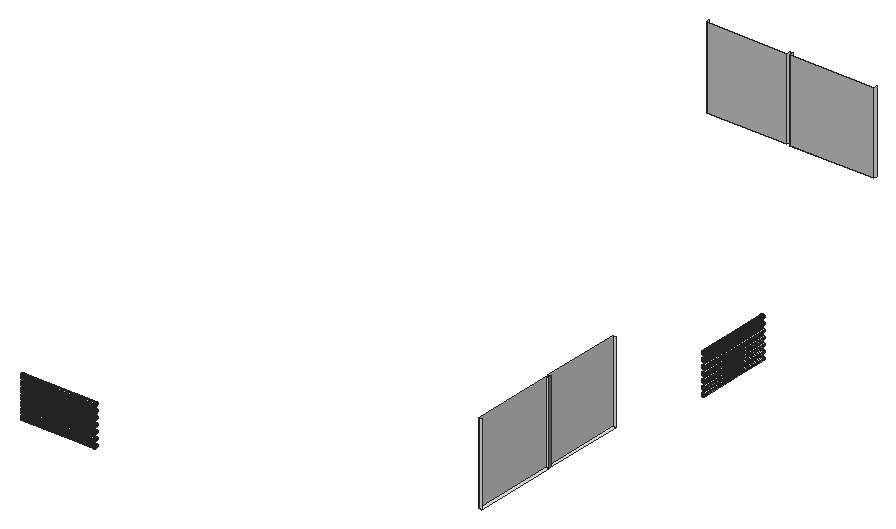
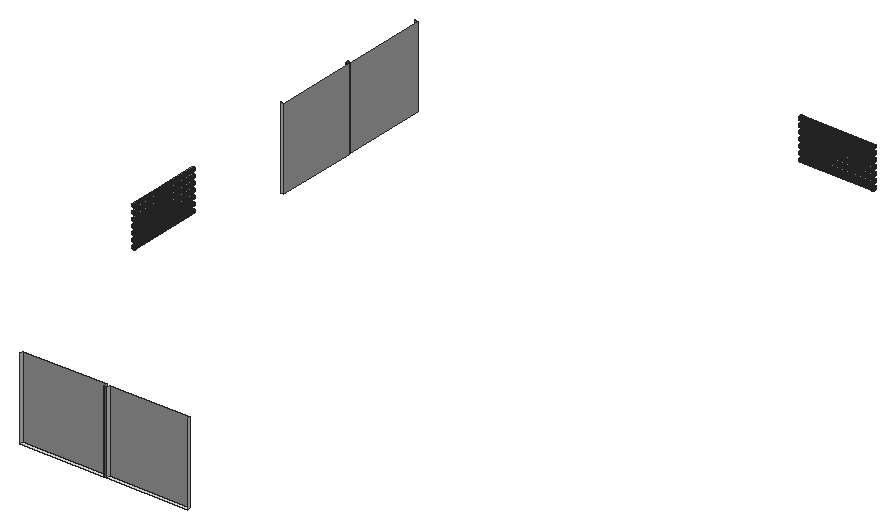
# SketchUp Ruby script. Lengths in inches.
U = 1.inch
M = Sketchup.active_model
def pt(a) = Geom::Point3d.new(a.map { |v| v * U })
def face(e, loops, mat)
  f = e.add_face(loops[0].map { |a| pt(a) })
  loops[1..].each { |l| e.add_face(l.map { |a| pt(a) }).erase! }
  f.material = f.back_material = mat if mat
  f
end
# faces: each face lists its corners as indices into pts; further lists are holes
def faces(e, pts, list, mat = nil) = list.each { |f| face(e, (f[0].is_a?(Array) ? f : [f]).map { |l| l.map { |i| pts[i] } }, mat) }
# xy, xz, yz: faces in a plane at the given z, y or x. An outline is a flat list of corners, or four numbers for a rectangle; further outlines are holes
def ring(l) = l.size == 4 ? [[l[0], l[1]], [l[2], l[1]], [l[2], l[3]], [l[0], l[3]]] : l.each_slice(2).to_a
def flat(e, list, mat, &to3) = list.each { |f| face(e, (f[0].is_a?(Array) ? f : [f]).map { |l| ring(l).map { |u, v| to3.(u, v) } }, mat) }
def xy(e, z, list, mat = nil) = flat(e, list, mat) { |x, y| [x, y, z] }
def xz(e, y, list, mat = nil) = flat(e, list, mat) { |x, z| [x, y, z] }
def yz(e, x, list, mat = nil) = flat(e, list, mat) { |y, z| [x, y, z] }
def lines(e, pts, list) = list.each { |a, b| e.add_line(pt(pts[a]), pt(pts[b])) }
# prism: a flat outline (further loops are holes) pulled along v
def prism(e, loops, v, mat = nil)
  f = face(e, loops, mat); d = Geom::Vector3d.new(v.map { |x| x * U })
  f.pushpull(f.normal.samedirection?(d) ? d.length : -d.length)
end
def box(e, o, s, mat = nil) = prism(e, [[o, [o[0] + s[0], o[1], o[2]], [o[0] + s[0], o[1] + s[1], o[2]], [o[0], o[1] + s[1], o[2]]]], [0, 0, s[2]], mat)
def at(x, y, z, deg = 0) = Geom::Transformation.translation(pt([x, y, z])) * Geom::Transformation.rotation(ORIGIN, Z_AXIS, deg.degrees)
def axes(o, x, y, z) = Geom::Transformation.new([*x, 0, *y, 0, *z, 0, *pt(o).to_a, 1])
def part(name) = M.definitions.add(name)
# library, detail: a bought-in or finely detailed component or shape, given as its bounding box
def library(name, o, s) = part(name).tap { |d| box(d.entities, o, s) }
def detail(e, o, s) = box(e.add_group.entities, o, s)
def put(e, d, t, mat = nil) = e.add_instance(d, t).tap { |i| i.material = mat if mat }
def group(e, t, mat = nil) = e.add_group.tap { |g| g.transformation = t; g.material = mat if mat }.entities
root = M.entities
M.materials.add("[Metal Seamed]").color = [118, 119, 115]
M.materials.add("[Mirror 01]").color = [185, 185, 185]
xy(root,539.76,[[1476,277.47,1482,438.75],[1476,444.75,1482,600.03],[984.78,1440.8125,1140.0625,1446.8125],[1146.0625,1440.8125,1307.35,1446.8125]])
xz(root,277.47,[[1476,539.76,1482,696.625]])
xz(root,438.75,[[1476,539.76,1482,696.625]])
xz(root,444.75,[[1476,539.76,1482,696.625]])
xz(root,600.03,[[1476,539.76,1482,696.625]])
xz(root,1440.8125,[[984.78,539.76,1140.0625,696.625],[1146.0625,539.76,1307.35,696.625]],"[Mirror 01]")
xz(root,1446.8125,[[1140.0625,539.76,1146.0625,696.625]],"[Metal Seamed]")
yz(root,984.78,[[1440.8125,539.76,1446.8125,696.625]])
yz(root,1140.0625,[[1440.8125,539.76,1446.8125,696.625]])
yz(root,1146.0625,[[1440.8125,539.76,1446.8125,696.625]])
yz(root,1307.35,[[1440.8125,539.76,1446.8125,696.625]])
yz(root,1476,[[277.47,539.76,438.75,696.625],[444.75,539.76,600.03,696.625]],"[Mirror 01]")
yz(root,1482,[[438.75,539.76,444.75,696.625]],"[Metal Seamed]")
p = [[922.01,48.34,549.02],[922.01,47.38,549.14],[778.64,47.38,549.14],[778.64,48.34,549.02],[922.01,49.29,549.14],[778.64,49.29,549.14],
  [1535.52,886.83,549.14],[1536.47,886.83,549.02],[1536.47,743.45,549.02],[1535.52,743.45,549.14],[1537.43,886.83,549.14],[1537.43,743.45,549.14],
  [922.01,46.5,549.51],[778.64,46.5,549.51],[922.01,50.18,549.51],[778.64,50.18,549.51],[1534.63,886.83,549.51],[1534.63,743.45,549.51],
  [1538.32,886.83,549.51],[1538.32,743.45,549.51],[922.01,45.73,550.1],[778.64,45.73,550.1],[922.01,50.95,550.1],[778.64,50.95,550.1],
  [1533.87,886.83,550.1],[1533.87,743.45,550.1],[1539.08,886.83,550.1],[1539.08,743.45,550.1],[922.01,45.15,550.86],[778.64,45.15,550.86],
  [922.01,51.53,550.86],[778.64,51.53,550.86],[1533.28,886.83,550.86],[1533.28,743.45,550.86],[1539.67,886.83,550.86],[1539.67,743.45,550.86],
  [922.01,44.78,551.75],[778.64,44.78,551.75],[922.01,51.9,551.75],[778.64,51.9,551.75],[1532.91,886.83,551.75],[1532.91,743.45,551.75],
  [1540.03,886.83,551.75],[1540.03,743.45,551.75],[922.01,44.65,552.7],[778.64,44.65,552.7],[922.01,52.03,552.7],[778.64,52.03,552.7],
  [1532.79,886.83,552.7],[1532.79,743.45,552.7],[1540.16,886.83,552.7],[1540.16,743.45,552.7],[922.01,44.78,553.66],[778.64,44.78,553.66],
  [922.01,51.9,553.66],[778.64,51.9,553.66],[1532.91,886.83,553.66],[1532.91,743.45,553.66],[1540.03,886.83,553.66],[1540.03,743.45,553.66],
  [922.01,45.15,554.55],[778.64,45.15,554.55],[922.01,51.53,554.55],[778.64,51.53,554.55],[1533.28,886.83,554.55],[1533.28,743.45,554.55],
  [1539.67,886.83,554.55],[1539.67,743.45,554.55],[922.01,45.73,555.3125],[778.64,45.73,555.3125],[922.01,50.95,555.3125],[778.64,50.95,555.3125],
  [1533.87,886.83,555.3125],[1533.87,743.45,555.3125],[1539.08,886.83,555.3125],[1539.08,743.45,555.3125],[922.01,46.5,555.9],[778.64,46.5,555.9],
  [922.01,50.18,555.9],[778.64,50.18,555.9],[1534.63,886.83,555.9],[1534.63,743.45,555.9],[1538.32,886.83,555.9],[1538.32,743.45,555.9],
  [922.01,47.38,556.27],[778.64,47.38,556.27],[922.01,49.29,556.27],[778.64,49.29,556.27],[1535.52,886.83,556.27],[1535.52,743.45,556.27],
  [1537.43,886.83,556.27],[1537.43,743.45,556.27],[922.01,48.34,556.39],[778.64,48.34,556.39],[1536.47,886.83,556.39],[1536.47,743.45,556.39],
  [922.01,48.34,561.02],[922.01,47.38,561.14],[778.64,47.38,561.14],[778.64,48.34,561.02],[922.01,49.29,561.14],[778.64,49.29,561.14],
  [1535.52,886.83,561.14],[1536.47,886.83,561.02],[1536.47,743.45,561.02],[1535.52,743.45,561.14],[1537.43,886.83,561.14],[1537.43,743.45,561.14],
  [922.01,46.5,561.51],[778.64,46.5,561.51],[922.01,50.18,561.51],[778.64,50.18,561.51],[1534.63,886.83,561.51],[1534.63,743.45,561.51],
  [1538.32,886.83,561.51],[1538.32,743.45,561.51],[922.01,45.73,562.1],[778.64,45.73,562.1],[922.01,50.95,562.1],[778.64,50.95,562.1],
  [1533.87,886.83,562.1],[1533.87,743.45,562.1],[1539.08,886.83,562.1],[1539.08,743.45,562.1],[922.01,45.15,562.86],[778.64,45.15,562.86],
  [922.01,51.53,562.86],[778.64,51.53,562.86],[1533.28,886.83,562.86],[1533.28,743.45,562.86],[1539.67,886.83,562.86],[1539.67,743.45,562.86],
  [922.01,44.78,563.75],[778.64,44.78,563.75],[922.01,51.9,563.75],[778.64,51.9,563.75],[1532.91,886.83,563.75],[1532.91,743.45,563.75],
  [1540.03,886.83,563.75],[1540.03,743.45,563.75],[922.01,44.65,564.7],[778.64,44.65,564.7],[922.01,52.03,564.7],[778.64,52.03,564.7],
  [1532.79,886.83,564.7],[1532.79,743.45,564.7],[1540.16,886.83,564.7],[1540.16,743.45,564.7],[922.01,44.78,565.66],[778.64,44.78,565.66],
  [922.01,51.9,565.66],[778.64,51.9,565.66],[1532.91,886.83,565.66],[1532.91,743.45,565.66],[1540.03,886.83,565.66],[1540.03,743.45,565.66],
  [922.01,45.15,566.55],[778.64,45.15,566.55],[922.01,51.53,566.55],[778.64,51.53,566.55],[1533.28,886.83,566.55],[1533.28,743.45,566.55],
  [1539.67,886.83,566.55],[1539.67,743.45,566.55],[922.01,45.73,567.3125],[778.64,45.73,567.3125],[922.01,50.95,567.3125],[778.64,50.95,567.3125],
  [1533.87,886.83,567.3125],[1533.87,743.45,567.3125],[1539.08,886.83,567.3125],[1539.08,743.45,567.3125],[922.01,46.5,567.9],[778.64,46.5,567.9],
  [922.01,50.18,567.9],[778.64,50.18,567.9],[1534.63,886.83,567.9],[1534.63,743.45,567.9],[1538.32,886.83,567.9],[1538.32,743.45,567.9],
  [922.01,47.38,568.27],[778.64,47.38,568.27],[922.01,49.29,568.27],[778.64,49.29,568.27],[1535.52,886.83,568.27],[1535.52,743.45,568.27],
  [1537.43,886.83,568.27],[1537.43,743.45,568.27],[922.01,48.34,568.39],[778.64,48.34,568.39],[1536.47,886.83,568.39],[1536.47,743.45,568.39],
  [922.01,48.34,573.02],[922.01,47.38,573.14],[778.64,47.38,573.14],[778.64,48.34,573.02],[922.01,49.29,573.14],[778.64,49.29,573.14],
  [1535.52,886.83,573.14],[1536.47,886.83,573.02],[1536.47,743.45,573.02],[1535.52,743.45,573.14],[1537.43,886.83,573.14],[1537.43,743.45,573.14],
  [922.01,46.5,573.51],[778.64,46.5,573.51],[922.01,50.18,573.51],[778.64,50.18,573.51],[1534.63,886.83,573.51],[1534.63,743.45,573.51],
  [1538.32,886.83,573.51],[1538.32,743.45,573.51],[922.01,45.73,574.1],[778.64,45.73,574.1],[922.01,50.95,574.1],[778.64,50.95,574.1],
  [1533.87,886.83,574.1],[1533.87,743.45,574.1],[1539.08,886.83,574.1],[1539.08,743.45,574.1],[922.01,45.15,574.86],[778.64,45.15,574.86],
  [922.01,51.53,574.86],[778.64,51.53,574.86],[1533.28,886.83,574.86],[1533.28,743.45,574.86],[1539.67,886.83,574.86],[1539.67,743.45,574.86],
  [922.01,44.78,575.75],[778.64,44.78,575.75],[922.01,51.9,575.75],[778.64,51.9,575.75],[1532.91,886.83,575.75],[1532.91,743.45,575.75],
  [1540.03,886.83,575.75],[1540.03,743.45,575.75],[922.01,44.65,576.7],[778.64,44.65,576.7],[922.01,52.03,576.7],[778.64,52.03,576.7],
  [1532.79,886.83,576.7],[1532.79,743.45,576.7],[1540.16,886.83,576.7],[1540.16,743.45,576.7],[922.01,44.78,577.66],[778.64,44.78,577.66],
  [922.01,51.9,577.66],[778.64,51.9,577.66],[1532.91,886.83,577.66],[1532.91,743.45,577.66],[1540.03,886.83,577.66],[1540.03,743.45,577.66],
  [922.01,45.15,578.55],[778.64,45.15,578.55],[922.01,51.53,578.55],[778.64,51.53,578.55],[1533.28,886.83,578.55],[1533.28,743.45,578.55],
  [1539.67,886.83,578.55],[1539.67,743.45,578.55],[922.01,45.73,579.3125],[778.64,45.73,579.3125],[922.01,50.95,579.3125],[778.64,50.95,579.3125],
  [1533.87,886.83,579.3125],[1533.87,743.45,579.3125],[1539.08,886.83,579.3125],[1539.08,743.45,579.3125],[922.01,46.5,579.9],[778.64,46.5,579.9],
  [922.01,50.18,579.9],[778.64,50.18,579.9],[1534.63,886.83,579.9],[1534.63,743.45,579.9],[1538.32,886.83,579.9],[1538.32,743.45,579.9],
  [922.01,47.38,580.27],[778.64,47.38,580.27],[922.01,49.29,580.27],[778.64,49.29,580.27],[1535.52,886.83,580.27],[1535.52,743.45,580.27],
  [1537.43,886.83,580.27],[1537.43,743.45,580.27],[922.01,48.34,580.39],[778.64,48.34,580.39],[1536.47,886.83,580.39],[1536.47,743.45,580.39],
  [922.01,48.34,585.02],[922.01,47.38,585.14],[778.64,47.38,585.14],[778.64,48.34,585.02],[922.01,49.29,585.14],[778.64,49.29,585.14],
  [1535.52,886.83,585.14],[1536.47,886.83,585.02],[1536.47,743.45,585.02],[1535.52,743.45,585.14],[1537.43,886.83,585.14],[1537.43,743.45,585.14],
  [922.01,46.5,585.51],[778.64,46.5,585.51],[922.01,50.18,585.51],[778.64,50.18,585.51],[1534.63,886.83,585.51],[1534.63,743.45,585.51],
  [1538.32,886.83,585.51],[1538.32,743.45,585.51],[922.01,45.73,586.1],[778.64,45.73,586.1],[922.01,50.95,586.1],[778.64,50.95,586.1],
  [1533.87,886.83,586.1],[1533.87,743.45,586.1],[1539.08,886.83,586.1],[1539.08,743.45,586.1],[922.01,45.15,586.86],[778.64,45.15,586.86],
  [922.01,51.53,586.86],[778.64,51.53,586.86],[1533.28,886.83,586.86],[1533.28,743.45,586.86],[1539.67,886.83,586.86],[1539.67,743.45,586.86],
  [922.01,44.78,587.75],[778.64,44.78,587.75],[922.01,51.9,587.75],[778.64,51.9,587.75],[1532.91,886.83,587.75],[1532.91,743.45,587.75],
  [1540.03,886.83,587.75],[1540.03,743.45,587.75],[922.01,44.65,588.7],[778.64,44.65,588.7],[922.01,52.03,588.7],[778.64,52.03,588.7],
  [1532.79,886.83,588.7],[1532.79,743.45,588.7],[1540.16,886.83,588.7],[1540.16,743.45,588.7],[922.01,44.78,589.66],[778.64,44.78,589.66],
  [922.01,51.9,589.66],[778.64,51.9,589.66],[1532.91,886.83,589.66],[1532.91,743.45,589.66],[1540.03,886.83,589.66],[1540.03,743.45,589.66],
  [922.01,45.15,590.55],[778.64,45.15,590.55],[922.01,51.53,590.55],[778.64,51.53,590.55],[1533.28,886.83,590.55],[1533.28,743.45,590.55],
  [1539.67,886.83,590.55],[1539.67,743.45,590.55],[922.01,45.73,591.3125],[778.64,45.73,591.3125],[922.01,50.95,591.3125],[778.64,50.95,591.3125],
  [1533.87,886.83,591.3125],[1533.87,743.45,591.3125],[1539.08,886.83,591.3125],[1539.08,743.45,591.3125],[922.01,46.5,591.9],[778.64,46.5,591.9],
  [922.01,50.18,591.9],[778.64,50.18,591.9],[1534.63,886.83,591.9],[1534.63,743.45,591.9],[1538.32,886.83,591.9],[1538.32,743.45,591.9],
  [922.01,47.38,592.27],[778.64,47.38,592.27],[922.01,49.29,592.27],[778.64,49.29,592.27],[1535.52,886.83,592.27],[1535.52,743.45,592.27],
  [1537.43,886.83,592.27],[1537.43,743.45,592.27],[922.01,48.34,592.39],[778.64,48.34,592.39],[1536.47,886.83,592.39],[1536.47,743.45,592.39],
  [922.01,48.34,597.02],[922.01,47.38,597.14],[778.64,47.38,597.14],[778.64,48.34,597.02],[922.01,49.29,597.14],[778.64,49.29,597.14],
  [1535.52,886.83,597.14],[1536.47,886.83,597.02],[1536.47,743.45,597.02],[1535.52,743.45,597.14],[1537.43,886.83,597.14],[1537.43,743.45,597.14],
  [922.01,46.5,597.51],[778.64,46.5,597.51],[922.01,50.18,597.51],[778.64,50.18,597.51],[1534.63,886.83,597.51],[1534.63,743.45,597.51],
  [1538.32,886.83,597.51],[1538.32,743.45,597.51],[922.01,45.73,598.1],[778.64,45.73,598.1],[922.01,50.95,598.1],[778.64,50.95,598.1],
  [1533.87,886.83,598.1],[1533.87,743.45,598.1],[1539.08,886.83,598.1],[1539.08,743.45,598.1],[922.01,45.15,598.86],[778.64,45.15,598.86],
  [922.01,51.53,598.86],[778.64,51.53,598.86],[1533.28,886.83,598.86],[1533.28,743.45,598.86],[1539.67,886.83,598.86],[1539.67,743.45,598.86],
  [922.01,44.78,599.75],[778.64,44.78,599.75],[922.01,51.9,599.75],[778.64,51.9,599.75],[1532.91,886.83,599.75],[1532.91,743.45,599.75],
  [1540.03,886.83,599.75],[1540.03,743.45,599.75],[922.01,44.65,600.7],[778.64,44.65,600.7],[922.01,52.03,600.7],[778.64,52.03,600.7],
  [1532.79,886.83,600.7],[1532.79,743.45,600.7],[1540.16,886.83,600.7],[1540.16,743.45,600.7],[922.01,44.78,601.66],[778.64,44.78,601.66],
  [922.01,51.9,601.66],[778.64,51.9,601.66],[1532.91,886.83,601.66],[1532.91,743.45,601.66],[1540.03,886.83,601.66],[1540.03,743.45,601.66],
  [922.01,45.15,602.55],[778.64,45.15,602.55],[922.01,51.53,602.55],[778.64,51.53,602.55],[1533.28,886.83,602.55],[1533.28,743.45,602.55],
  [1539.67,886.83,602.55],[1539.67,743.45,602.55],[922.01,45.73,603.3125],[778.64,45.73,603.3125],[922.01,50.95,603.3125],[778.64,50.95,603.3125],
  [1533.87,886.83,603.3125],[1533.87,743.45,603.3125],[1539.08,886.83,603.3125],[1539.08,743.45,603.3125],[922.01,46.5,603.9],[778.64,46.5,603.9],
  [922.01,50.18,603.9],[778.64,50.18,603.9],[1534.63,886.83,603.9],[1534.63,743.45,603.9],[1538.32,886.83,603.9],[1538.32,743.45,603.9],
  [922.01,47.38,604.27],[778.64,47.38,604.27],[922.01,49.29,604.27],[778.64,49.29,604.27],[1535.52,886.83,604.27],[1535.52,743.45,604.27],
  [1537.43,886.83,604.27],[1537.43,743.45,604.27],[922.01,48.34,604.39],[778.64,48.34,604.39],[1536.47,886.83,604.39],[1536.47,743.45,604.39],
  [922.01,48.34,609.02],[922.01,47.38,609.14],[778.64,47.38,609.14],[778.64,48.34,609.02],[922.01,49.29,609.14],[778.64,49.29,609.14],
  [1535.52,886.83,609.14],[1536.47,886.83,609.02],[1536.47,743.45,609.02],[1535.52,743.45,609.14],[1537.43,886.83,609.14],[1537.43,743.45,609.14],
  [922.01,46.5,609.51],[778.64,46.5,609.51],[922.01,50.18,609.51],[778.64,50.18,609.51],[1534.63,886.83,609.51],[1534.63,743.45,609.51],
  [1538.32,886.83,609.51],[1538.32,743.45,609.51],[922.01,45.73,610.1],[778.64,45.73,610.1],[922.01,50.95,610.1],[778.64,50.95,610.1],
  [1533.87,886.83,610.1],[1533.87,743.45,610.1],[1539.08,886.83,610.1],[1539.08,743.45,610.1],[922.01,45.15,610.86],[778.64,45.15,610.86],
  [922.01,51.53,610.86],[778.64,51.53,610.86],[1533.28,886.83,610.86],[1533.28,743.45,610.86],[1539.67,886.83,610.86],[1539.67,743.45,610.86],
  [922.01,44.78,611.75],[778.64,44.78,611.75],[922.01,51.9,611.75],[778.64,51.9,611.75],[1532.91,886.83,611.75],[1532.91,743.45,611.75],
  [1540.03,886.83,611.75],[1540.03,743.45,611.75],[922.01,44.65,612.7],[778.64,44.65,612.7],[922.01,52.03,612.7],[778.64,52.03,612.7],
  [1532.79,886.83,612.7],[1532.79,743.45,612.7],[1540.16,886.83,612.7],[1540.16,743.45,612.7],[922.01,44.78,613.66],[778.64,44.78,613.66],
  [922.01,51.9,613.66],[778.64,51.9,613.66],[1532.91,886.83,613.66],[1532.91,743.45,613.66],[1540.03,886.83,613.66],[1540.03,743.45,613.66],
  [922.01,45.15,614.55],[778.64,45.15,614.55],[922.01,51.53,614.55],[778.64,51.53,614.55],[1533.28,886.83,614.55],[1533.28,743.45,614.55],
  [1539.67,886.83,614.55],[1539.67,743.45,614.55],[922.01,45.73,615.3125],[778.64,45.73,615.3125],[922.01,50.95,615.3125],[778.64,50.95,615.3125],
  [1533.87,886.83,615.3125],[1533.87,743.45,615.3125],[1539.08,886.83,615.3125],[1539.08,743.45,615.3125],[922.01,46.5,615.9],[778.64,46.5,615.9],
  [922.01,50.18,615.9],[778.64,50.18,615.9],[1534.63,886.83,615.9],[1534.63,743.45,615.9],[1538.32,886.83,615.9],[1538.32,743.45,615.9],
  [922.01,47.38,616.27],[778.64,47.38,616.27],[922.01,49.29,616.27],[778.64,49.29,616.27],[1535.52,886.83,616.27],[1535.52,743.45,616.27],
  [1537.43,886.83,616.27],[1537.43,743.45,616.27],[922.01,48.34,616.39],[778.64,48.34,616.39],[1536.47,886.83,616.39],[1536.47,743.45,616.39],
  [922.01,48.34,621.02],[922.01,47.38,621.14],[778.64,47.38,621.14],[778.64,48.34,621.02],[922.01,49.29,621.14],[778.64,49.29,621.14],
  [1535.52,886.83,621.14],[1536.47,886.83,621.02],[1536.47,743.45,621.02],[1535.52,743.45,621.14],[1537.43,886.83,621.14],[1537.43,743.45,621.14],
  [922.01,46.5,621.51],[778.64,46.5,621.51],[922.01,50.18,621.51],[778.64,50.18,621.51],[1534.63,886.83,621.51],[1534.63,743.45,621.51],
  [1538.32,886.83,621.51],[1538.32,743.45,621.51],[922.01,45.73,622.1],[778.64,45.73,622.1],[922.01,50.95,622.1],[778.64,50.95,622.1],
  [1533.87,886.83,622.1],[1533.87,743.45,622.1],[1539.08,886.83,622.1],[1539.08,743.45,622.1],[922.01,45.15,622.86],[778.64,45.15,622.86],
  [922.01,51.53,622.86],[778.64,51.53,622.86],[1533.28,886.83,622.86],[1533.28,743.45,622.86],[1539.67,886.83,622.86],[1539.67,743.45,622.86],
  [922.01,44.78,623.75],[778.64,44.78,623.75],[922.01,51.9,623.75],[778.64,51.9,623.75],[1532.91,886.83,623.75],[1532.91,743.45,623.75],
  [1540.03,886.83,623.75],[1540.03,743.45,623.75],[922.01,44.65,624.7],[778.64,44.65,624.7],[922.01,52.03,624.7],[778.64,52.03,624.7],
  [1532.79,886.83,624.7],[1532.79,743.45,624.7],[1540.16,886.83,624.7],[1540.16,743.45,624.7],[922.01,44.78,625.66],[778.64,44.78,625.66],
  [922.01,51.9,625.66],[778.64,51.9,625.66],[1532.91,886.83,625.66],[1532.91,743.45,625.66],[1540.03,886.83,625.66],[1540.03,743.45,625.66],
  [922.01,45.15,626.55],[778.64,45.15,626.55],[922.01,51.53,626.55],[778.64,51.53,626.55],[1533.28,886.83,626.55],[1533.28,743.45,626.55],
  [1539.67,886.83,626.55],[1539.67,743.45,626.55],[922.01,45.73,627.3125],[778.64,45.73,627.3125],[922.01,50.95,627.3125],[778.64,50.95,627.3125],
  [1533.87,886.83,627.3125],[1533.87,743.45,627.3125],[1539.08,886.83,627.3125],[1539.08,743.45,627.3125],[922.01,46.5,627.9],[778.64,46.5,627.9],
  [922.01,50.18,627.9],[778.64,50.18,627.9],[1534.63,886.83,627.9],[1534.63,743.45,627.9],[1538.32,886.83,627.9],[1538.32,743.45,627.9],
  [922.01,47.38,628.27],[778.64,47.38,628.27],[922.01,49.29,628.27],[778.64,49.29,628.27],[1535.52,886.83,628.27],[1535.52,743.45,628.27],
  [1537.43,886.83,628.27],[1537.43,743.45,628.27],[922.01,48.34,628.39],[778.64,48.34,628.39],[1536.47,886.83,628.39],[1536.47,743.45,628.39]]
faces(root,p,[[0,1,2,3],[4,0,3,5],[6,7,8,9],[7,10,11,8],[1,12,13,2],[14,4,5,15],[16,6,9,17],[10,18,19,11],
  [12,20,21,13],[22,14,15,23],[24,16,17,25],[18,26,27,19],[20,28,29,21],[30,22,23,31],[32,24,25,33],[26,34,35,27],
  [28,36,37,29],[38,30,31,39],[40,32,33,41],[34,42,43,35],[36,44,45,37],[46,38,39,47],[48,40,41,49],[42,50,51,43],
  [44,52,53,45],[54,46,47,55],[56,48,49,57],[50,58,59,51],[52,60,61,53],[62,54,55,63],[64,56,57,65],[58,66,67,59],
  [60,68,69,61],[70,62,63,71],[72,64,65,73],[66,74,75,67],[68,76,77,69],[78,70,71,79],[80,72,73,81],[74,82,83,75],
  [76,84,85,77],[86,78,79,87],[88,80,81,89],[82,90,91,83],[84,92,93,85],[92,86,87,93],[94,88,89,95],[90,94,95,91],
  [96,97,98,99],[100,96,99,101],[102,103,104,105],[103,106,107,104],[97,108,109,98],[110,100,101,111],[112,102,105,113],[106,114,115,107],
  [108,116,117,109],[118,110,111,119],[120,112,113,121],[114,122,123,115],[116,124,125,117],[126,118,119,127],[128,120,121,129],[122,130,131,123],
  [124,132,133,125],[134,126,127,135],[136,128,129,137],[130,138,139,131],[132,140,141,133],[142,134,135,143],[144,136,137,145],[138,146,147,139],
  [140,148,149,141],[150,142,143,151],[152,144,145,153],[146,154,155,147],[148,156,157,149],[158,150,151,159],[160,152,153,161],[154,162,163,155],
  [156,164,165,157],[166,158,159,167],[168,160,161,169],[162,170,171,163],[164,172,173,165],[174,166,167,175],[176,168,169,177],[170,178,179,171],
  [172,180,181,173],[182,174,175,183],[184,176,177,185],[178,186,187,179],[180,188,189,181],[188,182,183,189],[190,184,185,191],[186,190,191,187],
  [192,193,194,195],[196,192,195,197],[198,199,200,201],[199,202,203,200],[193,204,205,194],[206,196,197,207],[208,198,201,209],[202,210,211,203],
  [204,212,213,205],[214,206,207,215],[216,208,209,217],[210,218,219,211],[212,220,221,213],[222,214,215,223],[224,216,217,225],[218,226,227,219],
  [220,228,229,221],[230,222,223,231],[232,224,225,233],[226,234,235,227],[228,236,237,229],[238,230,231,239],[240,232,233,241],[234,242,243,235],
  [236,244,245,237],[246,238,239,247],[248,240,241,249],[242,250,251,243],[244,252,253,245],[254,246,247,255],[256,248,249,257],[250,258,259,251],
  [252,260,261,253],[262,254,255,263],[264,256,257,265],[258,266,267,259],[260,268,269,261],[270,262,263,271],[272,264,265,273],[266,274,275,267],
  [268,276,277,269],[278,270,271,279],[280,272,273,281],[274,282,283,275],[276,284,285,277],[284,278,279,285],[286,280,281,287],[282,286,287,283],
  [288,289,290,291],[292,288,291,293],[294,295,296,297],[295,298,299,296],[289,300,301,290],[302,292,293,303],[304,294,297,305],[298,306,307,299],
  [300,308,309,301],[310,302,303,311],[312,304,305,313],[306,314,315,307],[308,316,317,309],[318,310,311,319],[320,312,313,321],[314,322,323,315],
  [316,324,325,317],[326,318,319,327],[328,320,321,329],[322,330,331,323],[324,332,333,325],[334,326,327,335],[336,328,329,337],[330,338,339,331],
  [332,340,341,333],[342,334,335,343],[344,336,337,345],[338,346,347,339],[340,348,349,341],[350,342,343,351],[352,344,345,353],[346,354,355,347],
  [348,356,357,349],[358,350,351,359],[360,352,353,361],[354,362,363,355],[356,364,365,357],[366,358,359,367],[368,360,361,369],[362,370,371,363],
  [364,372,373,365],[374,366,367,375],[376,368,369,377],[370,378,379,371],[372,380,381,373],[380,374,375,381],[382,376,377,383],[378,382,383,379],
  [384,385,386,387],[388,384,387,389],[390,391,392,393],[391,394,395,392],[385,396,397,386],[398,388,389,399],[400,390,393,401],[394,402,403,395],
  [396,404,405,397],[406,398,399,407],[408,400,401,409],[402,410,411,403],[404,412,413,405],[414,406,407,415],[416,408,409,417],[410,418,419,411],
  [412,420,421,413],[422,414,415,423],[424,416,417,425],[418,426,427,419],[420,428,429,421],[430,422,423,431],[432,424,425,433],[426,434,435,427],
  [428,436,437,429],[438,430,431,439],[440,432,433,441],[434,442,443,435],[436,444,445,437],[446,438,439,447],[448,440,441,449],[442,450,451,443],
  [444,452,453,445],[454,446,447,455],[456,448,449,457],[450,458,459,451],[452,460,461,453],[462,454,455,463],[464,456,457,465],[458,466,467,459],
  [460,468,469,461],[470,462,463,471],[472,464,465,473],[466,474,475,467],[468,476,477,469],[476,470,471,477],[478,472,473,479],[474,478,479,475],
  [480,481,482,483],[484,480,483,485],[486,487,488,489],[487,490,491,488],[481,492,493,482],[494,484,485,495],[496,486,489,497],[490,498,499,491],
  [492,500,501,493],[502,494,495,503],[504,496,497,505],[498,506,507,499],[500,508,509,501],[510,502,503,511],[512,504,505,513],[506,514,515,507],
  [508,516,517,509],[518,510,511,519],[520,512,513,521],[514,522,523,515],[516,524,525,517],[526,518,519,527],[528,520,521,529],[522,530,531,523],
  [524,532,533,525],[534,526,527,535],[536,528,529,537],[530,538,539,531],[532,540,541,533],[542,534,535,543],[544,536,537,545],[538,546,547,539],
  [540,548,549,541],[550,542,543,551],[552,544,545,553],[546,554,555,547],[548,556,557,549],[558,550,551,559],[560,552,553,561],[554,562,563,555],
  [556,564,565,557],[566,558,559,567],[568,560,561,569],[562,570,571,563],[564,572,573,565],[572,566,567,573],[574,568,569,575],[570,574,575,571],
  [576,577,578,579],[580,576,579,581],[582,583,584,585],[583,586,587,584],[577,588,589,578],[590,580,581,591],[592,582,585,593],[586,594,595,587],
  [588,596,597,589],[598,590,591,599],[600,592,593,601],[594,602,603,595],[596,604,605,597],[606,598,599,607],[608,600,601,609],[602,610,611,603],
  [604,612,613,605],[614,606,607,615],[616,608,609,617],[610,618,619,611],[612,620,621,613],[622,614,615,623],[624,616,617,625],[618,626,627,619],
  [620,628,629,621],[630,622,623,631],[632,624,625,633],[626,634,635,627],[628,636,637,629],[638,630,631,639],[640,632,633,641],[634,642,643,635],
  [636,644,645,637],[646,638,639,647],[648,640,641,649],[642,650,651,643],[644,652,653,645],[654,646,647,655],[656,648,649,657],[650,658,659,651],
  [652,660,661,653],[662,654,655,663],[664,656,657,665],[658,666,667,659],[660,668,669,661],[668,662,663,669],[670,664,665,671],[666,670,671,667]])
